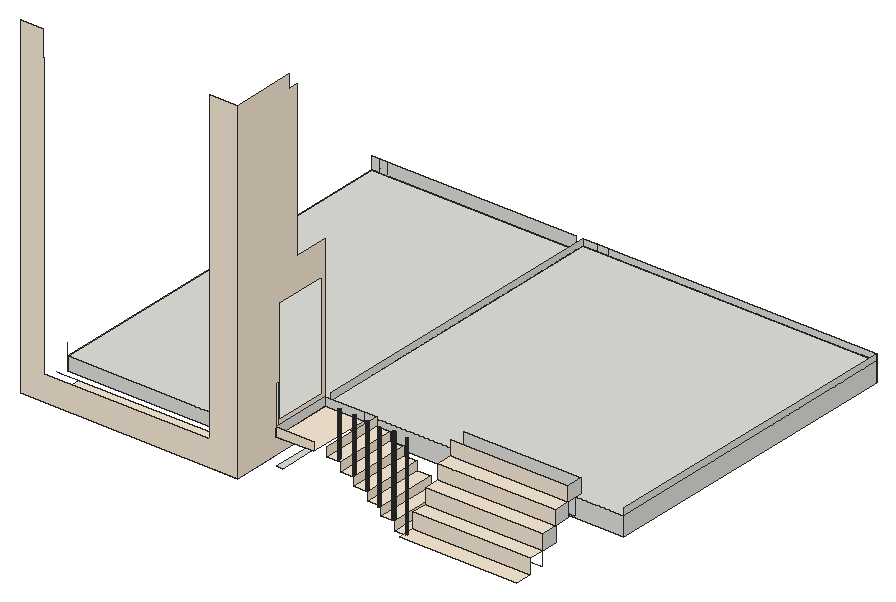
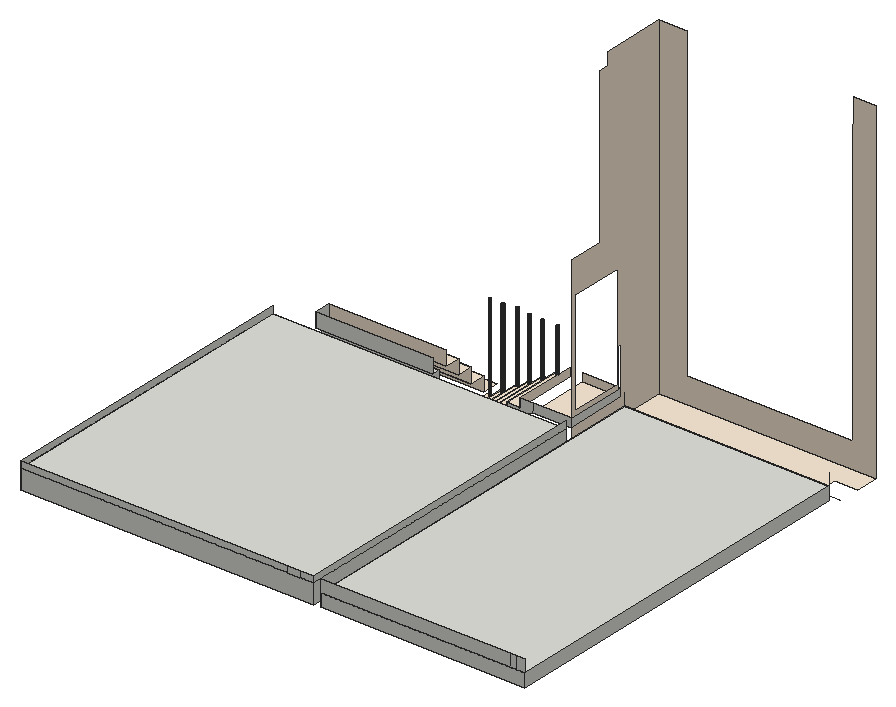
# SketchUp Ruby script. Lengths in inches.
U = 1.inch
M = Sketchup.active_model
def pt(a) = Geom::Point3d.new(a.map { |v| v * U })
def face(e, loops, mat)
  f = e.add_face(loops[0].map { |a| pt(a) })
  loops[1..].each { |l| e.add_face(l.map { |a| pt(a) }).erase! }
  f.material = f.back_material = mat if mat
  f
end
# faces: each face lists its corners as indices into pts; further lists are holes
def faces(e, pts, list, mat = nil) = list.each { |f| face(e, (f[0].is_a?(Array) ? f : [f]).map { |l| l.map { |i| pts[i] } }, mat) }
# xy, xz, yz: faces in a plane at the given z, y or x. An outline is a flat list of corners, or four numbers for a rectangle; further outlines are holes
def ring(l) = l.size == 4 ? [[l[0], l[1]], [l[2], l[1]], [l[2], l[3]], [l[0], l[3]]] : l.each_slice(2).to_a
def flat(e, list, mat, &to3) = list.each { |f| face(e, (f[0].is_a?(Array) ? f : [f]).map { |l| ring(l).map { |u, v| to3.(u, v) } }, mat) }
def xy(e, z, list, mat = nil) = flat(e, list, mat) { |x, y| [x, y, z] }
def xz(e, y, list, mat = nil) = flat(e, list, mat) { |x, z| [x, y, z] }
def yz(e, x, list, mat = nil) = flat(e, list, mat) { |y, z| [x, y, z] }
def lines(e, pts, list) = list.each { |a, b| e.add_line(pt(pts[a]), pt(pts[b])) }
# prism: a flat outline (further loops are holes) pulled along v
def prism(e, loops, v, mat = nil)
  f = face(e, loops, mat); d = Geom::Vector3d.new(v.map { |x| x * U })
  f.pushpull(f.normal.samedirection?(d) ? d.length : -d.length)
end
def box(e, o, s, mat = nil) = prism(e, [[o, [o[0] + s[0], o[1], o[2]], [o[0] + s[0], o[1] + s[1], o[2]], [o[0], o[1] + s[1], o[2]]]], [0, 0, s[2]], mat)
def at(x, y, z, deg = 0) = Geom::Transformation.translation(pt([x, y, z])) * Geom::Transformation.rotation(ORIGIN, Z_AXIS, deg.degrees)
def axes(o, x, y, z) = Geom::Transformation.new([*x, 0, *y, 0, *z, 0, *pt(o).to_a, 1])
def part(name) = M.definitions.add(name)
# library, detail: a bought-in or finely detailed component or shape, given as its bounding box
def library(name, o, s) = part(name).tap { |d| box(d.entities, o, s) }
def detail(e, o, s) = box(e.add_group.entities, o, s)
def put(e, d, t, mat = nil) = e.add_instance(d, t).tap { |i| i.material = mat if mat }
def group(e, t, mat = nil) = e.add_group.tap { |g| g.transformation = t; g.material = mat if mat }.entities
root = M.entities
M.materials.add("[0028_AntiqueWhite]").color = [250, 235, 215]
M.materials.add("[Color M08]").color = [30, 30, 30]
xy(root,129,[[[343.21,234.5,355.75,292.4375],[353.9,235.17,353.74,235.2,353.59,235.26,353.46,235.36,353.36,235.49,353.3,235.64,353.28,235.8,353.3,235.96,353.36,236.11,353.46,236.24,353.59,236.34,353.74,236.4,353.9,236.42,354.0625,236.4,354.21,236.34,354.34,236.24,354.44,236.11,354.5,235.96,354.53,235.8,354.5,235.64,354.44,235.49,354.34,235.36,354.21,235.26,354.0625,235.2]]],"[0028_AntiqueWhite]")
xy(root,129,[[353.9,235.17,353.74,235.2,353.59,235.26,353.46,235.36,353.36,235.49,353.3,235.64,353.28,235.8,353.3,235.96,353.36,236.11,353.46,236.24,353.59,236.34,353.74,236.4,353.9,236.42,354.0625,236.4,354.21,236.34,354.34,236.24,354.44,236.11,354.5,235.96,354.53,235.8,354.5,235.64,354.44,235.49,354.34,235.36,354.21,235.26,354.0625,235.2]],"[Color M08]")
xy(root,132.57,[[355.75,225.41,465.14,240.3]],"[0028_AntiqueWhite]")
xy(root,137,[[[330.68,234.5,343.21,292.4375],[341.03,235.41,340.71,235.45,340.41,235.58,340.15,235.77,339.95,236.03,339.83,236.34,339.78,236.66,339.83,236.98,339.95,237.28,340.15,237.54,340.41,237.74,340.71,237.87,341.03,237.91,341.36,237.87,341.66,237.74,341.92,237.54,342.12,237.28,342.24,236.98,342.28,236.66,342.24,236.34,342.12,236.03,341.92,235.77,341.66,235.58,341.36,235.45]]],"[0028_AntiqueWhite]")
xy(root,137,[[341.03,235.41,340.71,235.45,340.41,235.58,340.15,235.77,339.95,236.03,339.83,236.34,339.78,236.66,339.83,236.98,339.95,237.28,340.15,237.54,340.41,237.74,340.71,237.87,341.03,237.91,341.36,237.87,341.66,237.74,341.92,237.54,342.12,237.28,342.24,236.98,342.28,236.66,342.24,236.34,342.12,236.03,341.92,235.77,341.66,235.58,341.36,235.45]],"[Color M08]")
xy(root,138.45,[[226.3125,243.1,232.3125,283.98]])
xy(root,145,[[318.14,234.5,327.9,234.5,327.9,234.53,327.9375,234.86,328.0625,235.16,328.26,235.42,328.52,235.62,328.82,235.74,329.15,235.78,329.47,235.74,329.77,235.62,330.03,235.42,330.23,235.16,330.35,234.86,330.4,234.53,330.39,234.5,330.68,234.5,330.68,292.4375,318.14,292.4375]],"[0028_AntiqueWhite]")
xy(root,145,[[329.15,233.28,328.82,233.33,328.52,233.45,328.26,233.65,328.0625,233.91,327.9375,234.21,327.9,234.5,330.39,234.5,330.35,234.21,330.23,233.91,330.03,233.65,329.77,233.45,329.47,233.33],[327.9,234.5,327.9,234.53,327.9375,234.86,328.0625,235.16,328.26,235.42,328.52,235.62,328.82,235.74,329.15,235.78,329.47,235.74,329.77,235.62,330.03,235.42,330.23,235.16,330.35,234.86,330.4,234.53,330.39,234.5]],"[Color M08]")
xy(root,146.3,[[355.75,240.3,465.14,255.2]],"[0028_AntiqueWhite]")
xy(root,153,[[29.1875,190.5,29.1875,212.0625,50.75,212.0625,50.75,231.9375,232.3125,231.9375,232.3125,190.5],[[305.61,234.5,318.14,292.4375],[316.02,235.77,315.7,235.82,315.4,235.94,315.14,236.14,314.94,236.4,314.82,236.7,314.77,237.02,314.82,237.35,314.94,237.65,315.14,237.91,315.4,238.11,315.7,238.23,316.02,238.27,316.35,238.23,316.65,238.11,316.91,237.91,317.11,237.65,317.23,237.35,317.27,237.02,317.23,236.7,317.11,236.4,316.91,236.14,316.65,235.94,316.35,235.82]]],"[0028_AntiqueWhite]")
xy(root,153,[[316.02,235.77,315.7,235.82,315.4,235.94,315.14,236.14,314.94,236.4,314.82,236.7,314.77,237.02,314.82,237.35,314.94,237.65,315.14,237.91,315.4,238.11,315.7,238.23,316.02,238.27,316.35,238.23,316.65,238.11,316.91,237.91,317.11,237.65,317.23,237.35,317.27,237.02,317.23,236.7,317.11,236.4,316.91,236.14,316.65,235.94,316.35,235.82]],"[Color M08]")
xy(root,160.03,[[355.75,255.2,465.14,270.09]],"[0028_AntiqueWhite]")
xy(root,161,[[[293.07,234.5,305.61,292.4375],[303.28,236.26,302.95,236.31,302.65,236.43,302.39,236.63,302.19,236.89,302.07,237.19,302.03,237.51,302.07,237.84,302.19,238.14,302.39,238.4,302.65,238.6,302.95,238.72,303.28,238.76,303.6,238.72,303.9,238.6,304.16,238.4,304.36,238.14,304.48,237.84,304.53,237.51,304.48,237.19,304.36,236.89,304.16,236.63,303.9,236.43,303.6,236.31]]],"[0028_AntiqueWhite]")
xy(root,161,[[303.28,236.26,302.95,236.31,302.65,236.43,302.39,236.63,302.19,236.89,302.07,237.19,302.03,237.51,302.07,237.84,302.19,238.14,302.39,238.4,302.65,238.6,302.95,238.72,303.28,238.76,303.6,238.72,303.9,238.6,304.16,238.4,304.36,238.14,304.48,237.84,304.53,237.51,304.48,237.19,304.36,236.89,304.16,236.63,303.9,236.43,303.6,236.31]],"[Color M08]")
xy(root,165.3125,[[35.1875,237.9375,226.3125,592.9375]])
xy(root,169,[[232.3125,234.5,268,292.4375],[[280.54,234.5,293.07,292.4375],[289.3125,236.26,288.99,236.31,288.6875,236.43,288.43,236.63,288.23,236.89,288.1,237.19,288.0625,237.51,288.1,237.84,288.23,238.14,288.43,238.4,288.6875,238.6,288.99,238.72,289.3125,238.76,289.64,238.72,289.9375,238.6,290.2,238.4,290.39,238.14,290.52,237.84,290.5625,237.51,290.52,237.19,290.39,236.89,290.2,236.63,289.9375,236.43,289.64,236.31]]],"[0028_AntiqueWhite]")
xy(root,169,[[289.3125,236.26,288.99,236.31,288.6875,236.43,288.43,236.63,288.23,236.89,288.1,237.19,288.0625,237.51,288.1,237.84,288.23,238.14,288.43,238.4,288.6875,238.6,288.99,238.72,289.3125,238.76,289.64,238.72,289.9375,238.6,290.2,238.4,290.39,238.14,290.52,237.84,290.5625,237.51,290.52,237.19,290.39,236.89,290.2,236.63,289.9375,236.43,289.64,236.31]],"[Color M08]")
xy(root,171,[[232.3125,298.4375,506.4375,592.9375]])
xy(root,173.76,[[355.75,292.4375,465.14,299.89]])
xy(root,173.76,[[355.75,270.09,465.14,284.99]],"[0028_AntiqueWhite]")
xz(root,190.5,[[29.1875,153,232.3125,153,232.3125,465,206.3125,465,206.3125,441,206.5625,441,206.5625,177,50.75,177,50.75,297,50.7,297,50.7,321,50.75,321,50.75,441,50.63,441,50.63,465,29.1875,465]],"[0028_AntiqueWhite]")
xz(root,234.5,[[232.3125,169,268,177]],"[0028_AntiqueWhite]")
xz(root,237.9375,[[35.1875,153,226.3125,165.3125]])
xz(root,240.3,[[355.75,132.57,465.14,146.3]],"[0028_AntiqueWhite]")
xz(root,255.2,[[355.75,146.3,465.14,160.03]],"[0028_AntiqueWhite]")
xz(root,270.09,[[355.75,160.03,465.14,173.76]],"[0028_AntiqueWhite]")
xz(root,284.99,[[355.75,173.76,465.14,187.49]],"[0028_AntiqueWhite]")
xz(root,292.4375,[[294.56,153,305.61,153,305.61,161,293.07,161,293.07,169,280.54,169,280.54,177,268,177,268,169],[355.75,159.01,465.14,173.76],[232.3125,169,268,177]])
xz(root,298.4375,[[232.3125,153,506.4375,171]])
xz(root,299.89,[[355.75,173.76,465.14,187.49]])
xz(root,592.9375,[[35.1875,153,226.3125,165.3125],[232.3125,153,506.4375,171],[35.1875,165.3125,43.01,177],[43.01,165.3125,49.57,177],[49.57,165.3125,226.3125,177],
  [232.3125,171,245.32,177],[245.32,171,256.95,177],[256.95,171,506.4375,177]])
yz(root,35.1875,[[237.9375,153,592.9375,165.3125]])
yz(root,226.3125,[[237.9375,153,592.9375,165.3125]])
yz(root,232.3125,[[298.4375,153,592.9375,171],[234.5,169,292.4375,177],[298.4375,171,592.9375,177]])
yz(root,232.3125,[[[190.5,153,292.4375,153,292.4375,169,234.5,169,234.5,213,238.33,213,238.33,177,292.4375,177,292.4375,309,259.125,309,259.125,453,250.5,453,250.5,465,190.5,465],[238.8,181.1,288.24,278.41]]],"[0028_AntiqueWhite]")
yz(root,280.54,[[234.5,169,292.4375,177]],"[0028_AntiqueWhite]")
yz(root,293.07,[[234.5,161,292.4375,169]],"[0028_AntiqueWhite]")
yz(root,305.61,[[234.5,153,292.4375,161]],"[0028_AntiqueWhite]")
yz(root,318.14,[[234.5,145,292.4375,153]],"[0028_AntiqueWhite]")
yz(root,330.68,[[234.5,137,292.4375,145]],"[0028_AntiqueWhite]")
yz(root,343.21,[[234.5,129,292.4375,137]],"[0028_AntiqueWhite]")
yz(root,465.14,[[255.2,146.3,270.09,160.03],[270.09,160.03,284.99,173.76],[284.99,173.76,299.89,187.49]])
yz(root,506.4375,[[298.4375,153,592.9375,171],[298.4375,171,592.9375,177]])
p = [[353.59,235.26,129],[353.74,235.2,129],[353.74,235.2,209.625],[353.59,235.26,209.625],[353.9,235.17,129],[353.9,235.17,209.625],
  [354.0625,235.2,129],[354.0625,235.2,209.625],[354.21,235.26,129],[354.21,235.26,209.625],[353.46,235.36,129],[353.46,235.36,209.625],
  [354.34,235.36,129],[354.34,235.36,209.625],[353.36,235.49,129],[353.36,235.49,209.625],[354.44,235.49,129],[354.44,235.49,209.625],
  [353.3,235.64,129],[353.3,235.64,209.625],[354.5,235.64,129],[354.5,235.64,209.625],[353.28,235.8,129],[353.28,235.8,209.625],
  [354.53,235.8,129],[354.53,235.8,209.625],[353.3,235.96,129],[353.3,235.96,209.625],[354.5,235.96,129],[354.5,235.96,209.625],
  [353.36,236.11,129],[353.36,236.11,209.625],[354.44,236.11,129],[354.44,236.11,209.625],[353.46,236.24,129],[353.46,236.24,209.625],
  [354.34,236.24,129],[354.34,236.24,209.625],[353.59,236.34,129],[353.59,236.34,209.625],[354.21,236.34,129],[354.21,236.34,209.625],
  [353.74,236.4,129],[353.74,236.4,209.625],[354.0625,236.4,129],[354.0625,236.4,209.625],[353.9,236.42,129],[353.9,236.42,209.625],
  [340.71,235.45,137],[341.03,235.41,137],[341.03,235.41,209.97],[340.71,235.45,209.97],[341.36,235.45,137],[341.36,235.45,209.97],
  [340.41,235.58,137],[340.41,235.58,209.97],[341.66,235.58,137],[341.66,235.58,209.97],[340.15,235.77,137],[340.15,235.77,209.97],
  [341.92,235.77,137],[341.92,235.77,209.97],[339.95,236.03,137],[339.95,236.03,209.97],[342.12,236.03,137],[342.12,236.03,209.97],
  [339.83,236.34,137],[339.83,236.34,209.97],[342.24,236.34,137],[342.24,236.34,209.97],[339.78,236.66,137],[339.78,236.66,209.97],
  [342.28,236.66,137],[342.28,236.66,209.97],[339.83,236.98,137],[339.83,236.98,209.97],[342.24,236.98,137],[342.24,236.98,209.97],
  [339.95,237.28,137],[339.95,237.28,209.97],[342.12,237.28,137],[342.12,237.28,209.97],[340.15,237.54,137],[340.15,237.54,209.97],
  [341.92,237.54,137],[341.92,237.54,209.97],[340.41,237.74,137],[340.41,237.74,209.97],[341.66,237.74,137],[341.66,237.74,209.97],
  [340.71,237.87,137],[340.71,237.87,209.97],[341.36,237.87,137],[341.36,237.87,209.97],[341.03,237.91,137],[341.03,237.91,209.97],
  [328.52,233.45,145],[328.82,233.33,145],[328.82,233.33,209.97],[328.52,233.45,209.97],[329.15,233.28,145],[329.15,233.28,209.97],
  [329.47,233.33,145],[329.47,233.33,209.97],[329.77,233.45,145],[329.77,233.45,209.97],[328.26,233.65,145],[328.26,233.65,209.97],
  [330.03,233.65,145],[330.03,233.65,209.97],[328.0625,233.91,145],[328.0625,233.91,209.97],[330.23,233.91,145],[330.23,233.91,209.97],
  [327.9375,234.21,145],[327.9375,234.21,209.97],[330.35,234.21,145],[330.35,234.21,209.97],[327.9,234.5,145],[327.9,234.5,209.97],
  [327.9,234.53,209.97],[327.9,234.53,145],[330.39,234.5,145],[330.4,234.53,145],[330.4,234.53,209.97],[330.39,234.5,209.97],
  [327.9375,234.86,145],[327.9375,234.86,209.97],[330.35,234.86,145],[330.35,234.86,209.97],[328.0625,235.16,145],[328.0625,235.16,209.97],
  [330.23,235.16,145],[330.23,235.16,209.97],[328.26,235.42,145],[328.26,235.42,209.97],[330.03,235.42,145],[330.03,235.42,209.97],
  [328.52,235.62,145],[328.52,235.62,209.97],[329.77,235.62,145],[329.77,235.62,209.97],[328.82,235.74,145],[328.82,235.74,209.97],
  [329.47,235.74,145],[329.47,235.74,209.97],[329.15,235.78,145],[329.15,235.78,209.97],[315.4,235.94,153],[315.7,235.82,153],
  [315.7,235.82,209.97],[315.4,235.94,209.97],[316.02,235.77,153],[316.02,235.77,209.97],[316.35,235.82,153],[316.35,235.82,209.97],
  [316.65,235.94,153],[316.65,235.94,209.97],[315.14,236.14,153],[315.14,236.14,209.97],[316.91,236.14,153],[316.91,236.14,209.97],
  [314.94,236.4,153],[314.94,236.4,209.97],[317.11,236.4,153],[317.11,236.4,209.97],[314.82,236.7,153],[314.82,236.7,209.97],
  [317.23,236.7,153],[317.23,236.7,209.97],[314.77,237.02,153],[314.77,237.02,209.97],[317.27,237.02,153],[317.27,237.02,209.97],
  [314.82,237.35,153],[314.82,237.35,209.97],[317.23,237.35,153],[317.23,237.35,209.97],[314.94,237.65,153],[314.94,237.65,209.97],
  [317.11,237.65,153],[317.11,237.65,209.97],[315.14,237.91,153],[315.14,237.91,209.97],[316.91,237.91,153],[316.91,237.91,209.97],
  [315.4,238.11,153],[315.4,238.11,209.97],[316.65,238.11,153],[316.65,238.11,209.97],[315.7,238.23,153],[315.7,238.23,209.97],
  [316.35,238.23,153],[316.35,238.23,209.97],[316.02,238.27,153],[316.02,238.27,209.97],[302.65,236.43,161],[302.95,236.31,161],
  [302.95,236.31,209.97],[302.65,236.43,209.97],[303.28,236.26,161],[303.28,236.26,209.97],[303.6,236.31,161],[303.6,236.31,209.97],
  [303.9,236.43,161],[303.9,236.43,209.97],[302.39,236.63,161],[302.39,236.63,209.97],[304.16,236.63,161],[304.16,236.63,209.97],
  [302.19,236.89,161],[302.19,236.89,209.97],[304.36,236.89,161],[304.36,236.89,209.97],[302.07,237.19,161],[302.07,237.19,209.97],
  [304.48,237.19,161],[304.48,237.19,209.97],[302.03,237.51,161],[302.03,237.51,209.97],[304.53,237.51,161],[304.53,237.51,209.97],
  [302.07,237.84,161],[302.07,237.84,209.97],[304.48,237.84,161],[304.48,237.84,209.97],[302.19,238.14,161],[302.19,238.14,209.97],
  [304.36,238.14,161],[304.36,238.14,209.97],[302.39,238.4,161],[302.34,238.33,209.97],[302.39,238.4,209.97],[304.16,238.4,161],
  [304.16,238.4,209.97],[304.21,238.33,209.97],[302.65,238.6,161],[302.65,238.6,209.97],[303.9,238.6,161],[303.9,238.6,209.97],
  [302.95,238.72,161],[302.95,238.72,209.97],[303.6,238.72,161],[303.6,238.72,209.97],[303.28,238.76,161],[303.28,238.76,209.97],
  [288.6875,236.43,169],[288.99,236.31,169],[288.99,236.31,209.97],[288.6875,236.43,209.97],[289.3125,236.26,169],[289.3125,236.26,209.97],
  [289.64,236.31,169],[289.64,236.31,209.97],[289.9375,236.43,169],[289.9375,236.43,209.97],[288.43,236.63,169],[288.43,236.63,209.97],
  [290.2,236.63,169],[290.2,236.63,209.97],[288.23,236.89,169],[288.23,236.89,209.97],[290.39,236.89,169],[290.39,236.89,209.97],
  [288.1,237.19,169],[288.1,237.19,209.97],[290.52,237.19,169],[290.52,237.19,209.97],[288.0625,237.51,169],[288.0625,237.51,209.97],
  [290.5625,237.51,169],[290.5625,237.51,209.97],[288.1,237.84,169],[288.1,237.84,209.97],[290.52,237.84,169],[290.52,237.84,209.97],
  [288.23,238.14,169],[288.23,238.14,209.97],[290.39,238.14,169],[290.39,238.14,209.97],[288.43,238.4,169],[288.38,238.33,209.97],
  [288.43,238.4,209.97],[290.2,238.4,169],[290.2,238.4,209.97],[290.25,238.33,209.97],[288.6875,238.6,169],[288.6875,238.6,209.97],
  [289.9375,238.6,169],[289.9375,238.6,209.97],[288.99,238.72,169],[288.99,238.72,209.97],[289.64,238.72,169],[289.64,238.72,209.97],
  [289.3125,238.76,169],[289.3125,238.76,209.97],[29.1875,231.9375,153],[50.75,231.9375,153],[226.3125,237.9375,165.3125],[226.3125,237.9375,177],
  [35.1875,237.9375,165.3125],[35.1875,237.9375,177],[465.14,255.2,132.57],[465.14,255.2,146.3],[355.75,255.2,132.57]]
faces(root,p,[[0,1,2,3],[1,4,5,2],[4,6,7,5],[6,8,9,7],[10,0,3,11],[8,12,13,9],[14,10,11,15],[12,16,17,13],
  [18,14,15,19],[16,20,21,17],[22,18,19,23],[20,24,25,21],[26,22,23,27],[24,28,29,25],[30,26,27,31],[28,32,33,29],
  [34,30,31,35],[32,36,37,33],[38,34,35,39],[36,40,41,37],[42,38,39,43],[40,44,45,41],[46,42,43,47],[44,46,47,45],
  [48,49,50,51],[49,52,53,50],[54,48,51,55],[52,56,57,53],[58,54,55,59],[56,60,61,57],[62,58,59,63],[60,64,65,61],
  [66,62,63,67],[64,68,69,65],[70,66,67,71],[68,72,73,69],[74,70,71,75],[72,76,77,73],[78,74,75,79],[76,80,81,77],
  [82,78,79,83],[80,84,85,81],[86,82,83,87],[84,88,89,85],[90,86,87,91],[88,92,93,89],[94,90,91,95],[92,94,95,93],
  [96,97,98,99],[97,100,101,98],[100,102,103,101],[102,104,105,103],[106,96,99,107],[104,108,109,105],[110,106,107,111],[108,112,113,109],
  [114,110,111,115],[112,116,117,113],[118,114,115,119,120,121],[122,123,124,125,117,116],[126,121,120,127],[123,128,129,124],[130,126,127,131],[128,132,133,129],
  [134,130,131,135],[132,136,137,133],[138,134,135,139],[136,140,141,137],[142,138,139,143],[140,144,145,141],[146,142,143,147],[144,146,147,145],
  [148,149,150,151],[149,152,153,150],[152,154,155,153],[154,156,157,155],[158,148,151,159],[156,160,161,157],[162,158,159,163],[160,164,165,161],
  [166,162,163,167],[164,168,169,165],[170,166,167,171],[168,172,173,169],[174,170,171,175],[172,176,177,173],[178,174,175,179],[176,180,181,177],
  [182,178,179,183],[180,184,185,181],[186,182,183,187],[184,188,189,185],[190,186,187,191],[188,192,193,189],[194,190,191,195],[192,194,195,193],
  [196,197,198,199],[197,200,201,198],[200,202,203,201],[202,204,205,203],[206,196,199,207],[204,208,209,205],[210,206,207,211],[208,212,213,209],
  [214,210,211,215],[212,216,217,213],[218,214,215,219],[216,220,221,217],[222,218,219,223],[220,224,225,221],[226,222,223,227],[224,228,229,225],
  [230,226,227,231,232],[228,233,234,235,229],[236,230,232,237],[233,238,239,234],[240,236,237,241],[238,242,243,239],[244,240,241,245],[242,244,245,243],
  [246,247,248,249],[247,250,251,248],[250,252,253,251],[252,254,255,253],[256,246,249,257],[254,258,259,255],[260,256,257,261],[258,262,263,259],
  [264,260,261,265],[262,266,267,263],[268,264,265,269],[266,270,271,267],[272,268,269,273],[270,274,275,271],[276,272,273,277],[274,278,279,275],
  [280,276,277,281,282],[278,283,284,285,279],[286,280,282,287],[283,288,289,284],[290,286,287,291],[288,292,293,289],[294,290,291,295],[292,294,295,293]],"[Color M08]")
lines(root,p,[[296,297],[298,299],[300,301],[302,303],[304,302]])
